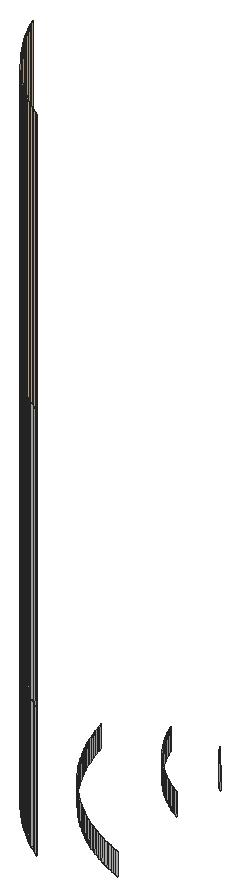
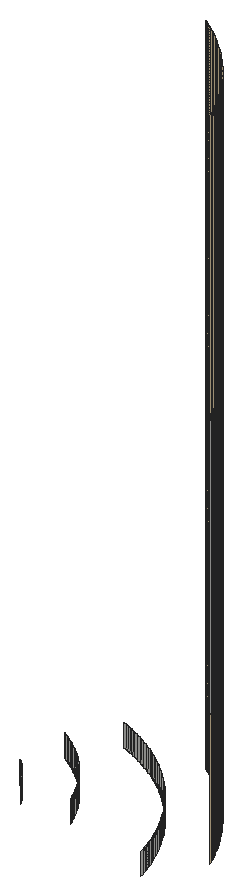
# SketchUp Ruby script. Lengths in inches.
U = 1.inch
M = Sketchup.active_model
def pt(a) = Geom::Point3d.new(a.map { |v| v * U })
def face(e, loops, mat)
  f = e.add_face(loops[0].map { |a| pt(a) })
  loops[1..].each { |l| e.add_face(l.map { |a| pt(a) }).erase! }
  f.material = f.back_material = mat if mat
  f
end
# faces: each face lists its corners as indices into pts; further lists are holes
def faces(e, pts, list, mat = nil) = list.each { |f| face(e, (f[0].is_a?(Array) ? f : [f]).map { |l| l.map { |i| pts[i] } }, mat) }
# xy, xz, yz: faces in a plane at the given z, y or x. An outline is a flat list of corners, or four numbers for a rectangle; further outlines are holes
def ring(l) = l.size == 4 ? [[l[0], l[1]], [l[2], l[1]], [l[2], l[3]], [l[0], l[3]]] : l.each_slice(2).to_a
def flat(e, list, mat, &to3) = list.each { |f| face(e, (f[0].is_a?(Array) ? f : [f]).map { |l| ring(l).map { |u, v| to3.(u, v) } }, mat) }
def xy(e, z, list, mat = nil) = flat(e, list, mat) { |x, y| [x, y, z] }
def xz(e, y, list, mat = nil) = flat(e, list, mat) { |x, z| [x, y, z] }
def yz(e, x, list, mat = nil) = flat(e, list, mat) { |y, z| [x, y, z] }
def lines(e, pts, list) = list.each { |a, b| e.add_line(pt(pts[a]), pt(pts[b])) }
# prism: a flat outline (further loops are holes) pulled along v
def prism(e, loops, v, mat = nil)
  f = face(e, loops, mat); d = Geom::Vector3d.new(v.map { |x| x * U })
  f.pushpull(f.normal.samedirection?(d) ? d.length : -d.length)
end
def box(e, o, s, mat = nil) = prism(e, [[o, [o[0] + s[0], o[1], o[2]], [o[0] + s[0], o[1] + s[1], o[2]], [o[0], o[1] + s[1], o[2]]]], [0, 0, s[2]], mat)
def at(x, y, z, deg = 0) = Geom::Transformation.translation(pt([x, y, z])) * Geom::Transformation.rotation(ORIGIN, Z_AXIS, deg.degrees)
def axes(o, x, y, z) = Geom::Transformation.new([*x, 0, *y, 0, *z, 0, *pt(o).to_a, 1])
def part(name) = M.definitions.add(name)
# library, detail: a bought-in or finely detailed component or shape, given as its bounding box
def library(name, o, s) = part(name).tap { |d| box(d.entities, o, s) }
def detail(e, o, s) = box(e.add_group.entities, o, s)
def put(e, d, t, mat = nil) = e.add_instance(d, t).tap { |i| i.material = mat if mat }
def group(e, t, mat = nil) = e.add_group.tap { |g| g.transformation = t; g.material = mat if mat }.entities
root = M.entities
M.materials.add("1026 AP 7946 SUNNY SIDE UP").color = [254, 231, 186]
p = [[23.33,229.02,252],[23.2,229.11,252],[23.2,229.11,246],[23.33,229.02,246],[23.36,229,246],[23.25,229.08,246],
  [23.25,229.08,276],[23.36,229,276],[23.15,229.15,246],[23.05,229.22,246],[23.05,229.22,276],[23.15,229.15,276],
  [23.07,229.2,252],[23.07,229.2,246],[22.95,229.29,246],[22.95,229.29,276],[22.95,229.29,252],[22.95,229.29,246],
  [22.85,229.37,246],[22.85,229.37,276],[22.82,229.38,252],[22.82,229.38,246],[22.74,229.44,246],[22.65,229.52,246],
  [22.65,229.52,276],[22.74,229.44,276],[22.69,229.48,252],[22.69,229.48,246],[22.55,229.6,246],[22.55,229.6,276],
  [22.57,229.58,252],[22.57,229.58,246],[22.45,229.67,246],[22.45,229.67,276],[22.45,229.67,252],[22.45,229.67,246],
  [26.54,229.62,246],[26.42,229.66,246],[26.42,229.66,247],[26.54,229.62,247],[22.33,229.77,252],[22.33,229.77,246],
  [22.35,229.75,246],[22.35,229.75,276],[26.29,229.71,246],[26.17,229.76,246],[26.17,229.76,247],[26.29,229.71,247],
  [22.25,229.83,246],[22.16,229.92,246],[22.16,229.92,276],[22.25,229.83,276],[22.21,229.875,252],[22.21,229.875,246],
  [26.05,229.8125,246],[25.93,229.86,246],[25.93,229.86,247],[26.05,229.8125,247],[22.0625,230,246],[22.0625,230,276],
  [22.09,229.98,252],[22.09,229.98,246],[25.8125,229.92,246],[25.69,229.97,246],[25.69,229.97,247],[25.8125,229.92,247],
  [21.97,230.08,246],[21.97,230.08,276],[21.97,230.08,252],[21.97,230.08,246],[25.58,230.03,246],[25.46,230.09,246],
  [25.46,230.09,247],[25.58,230.03,247],[21.88,230.17,246],[21.88,230.17,276],[21.85,230.1875,252],[21.85,230.1875,246],
  [25.34,230.15,246],[25.34,230.15,247],[21.74,230.3,252],[21.74,230.3,246],[21.79,230.25,246],[21.79,230.25,276],
  [25.23,230.21,246],[25.11,230.28,246],[25.11,230.28,247],[25.23,230.21,247],[21.69,230.34,246],[21.6,230.43,246],
  [21.6,230.43,276],[21.69,230.34,276],[21.625,230.4,252],[21.625,230.4,246],[25,230.34,246],[24.89,230.41,246],
  [24.89,230.41,247],[25,230.34,247],[21.51,230.51,246],[21.51,230.51,276],[21.51,230.51,252],[21.51,230.51,246],
  [24.78,230.47,246],[24.78,230.47,247],[21.43,230.6,246],[21.43,230.6,276],[21.4,230.625,252],[21.4,230.625,246],
  [24.66,230.54,246],[24.55,230.61,246],[24.55,230.61,247],[24.66,230.54,247],[21.34,230.69,246],[21.34,230.69,276],
  [21.3,230.74,252],[21.3,230.74,246],[24.44,230.69,246],[24.44,230.69,247],[21.1875,230.85,252],[21.1875,230.85,246],
  [21.25,230.79,246],[21.25,230.79,276],[24.34,230.76,246],[24.34,230.76,247],[21.17,230.88,246],[21.17,230.88,276],
  [24.23,230.83,246],[24.12,230.91,246],[24.12,230.91,247],[24.23,230.83,247],[21.08,230.97,246],[21.08,230.97,276],
  [21.08,230.97,252],[21.08,230.97,246],[24.02,230.99,246],[24.02,230.99,247],[21,231.0625,246],[21,231.0625,276],
  [20.98,231.09,252],[20.98,231.09,246],[23.91,231.07,246],[23.91,231.07,247],[20.92,231.16,246],[20.92,231.16,276],
  [20.875,231.21,252],[20.875,231.21,246],[23.81,231.15,246],[23.71,231.23,246],[23.71,231.23,247],[23.81,231.15,247],
  [20.83,231.25,246],[20.83,231.25,276],[20.77,231.33,252],[20.77,231.33,246],[23.61,231.3125,246],[23.61,231.3125,247],
  [20.67,231.45,252],[20.67,231.45,246],[20.75,231.35,246],[20.75,231.35,276],[23.51,231.4,246],[23.51,231.4,247],
  [20.67,231.45,246],[20.6,231.55,246],[20.6,231.55,276],[20.67,231.45,276],[20.58,231.57,252],[20.58,231.57,246],
  [23.41,231.48,246],[23.41,231.48,247],[20.52,231.65,246],[20.52,231.65,276],[23.31,231.57,246],[23.31,231.57,247],
  [20.44,231.74,246],[20.44,231.74,276],[20.48,231.69,252],[20.48,231.69,246],[23.21,231.66,246],[23.21,231.66,247],
  [20.37,231.85,246],[20.37,231.85,276],[20.38,231.82,252],[20.38,231.82,246],[23.12,231.75,246],[23.02,231.84,246],
  [23.02,231.84,247],[23.12,231.75,247],[20.29,231.95,246],[20.29,231.95,276],[20.29,231.95,252],[20.29,231.95,246],
  [22.93,231.93,246],[22.93,231.93,247],[20.22,232.05,246],[20.22,232.05,276],[20.2,232.07,252],[20.2,232.07,246],
  [22.84,232.02,246],[22.84,232.02,247],[20.15,232.15,246],[20.15,232.15,276],[22.75,232.12,246],[22.75,232.12,247],
  [20.11,232.2,252],[20.11,232.2,246],[22.66,232.21,246],[22.66,232.21,247],[20.02,232.33,252],[20.02,232.33,246],
  [20.08,232.25,246],[20.08,232.25,276],[22.57,232.31,246],[22.57,232.31,247],[19.9375,232.46,252],[19.9375,232.46,246],
  [20,232.36,246],[20,232.36,276],[22.48,232.41,246],[22.48,232.41,247],[19.9375,232.46,246],[19.9375,232.46,276],
  [22.4,232.51,246],[22.4,232.51,247],[19.87,232.57,246],[19.87,232.57,276],[19.85,232.6,252],[19.85,232.6,246],
  [22.3125,232.61,246],[22.3125,232.61,247],[19.8,232.68,246],[19.8,232.68,276],[19.77,232.73,252],[19.77,232.73,246],
  [22.23,232.71,246],[22.23,232.71,247],[19.74,232.78,246],[19.74,232.78,276],[19.6875,232.86,252],[19.6875,232.86,246],
  [22.15,232.81,246],[22.15,232.81,247],[19.67,232.89,246],[19.67,232.89,276],[22.07,232.91,246],[22.07,232.91,247],
  [19.61,233,246],[19.61,233,276],[19.61,233,252],[19.61,233,246],[21.99,233.02,246],[21.99,233.02,247],
  [19.55,233.11,246],[19.55,233.11,276],[19.53,233.14,252],[19.53,233.14,246],[21.91,233.12,246],[21.91,233.12,247],
  [19.48,233.22,246],[19.48,233.22,276],[19.45,233.27,252],[19.45,233.27,246],[21.83,233.23,246],[21.83,233.23,247],
  [19.42,233.33,246],[19.42,233.33,276],[21.76,233.34,246],[21.76,233.34,247],[19.37,233.44,246],[19.37,233.44,276],
  [19.38,233.41,252],[19.38,233.41,246],[21.69,233.44,246],[21.69,233.44,247],[19.31,233.55,246],[19.31,233.55,276],
  [19.31,233.55,252],[19.31,233.55,246],[21.61,233.55,246],[21.61,233.55,247],[19.24,233.69,252],[19.24,233.69,246],
  [19.25,233.66,246],[19.25,233.66,276],[21.54,233.66,246],[21.54,233.66,247],[19.2,233.78,246],[19.2,233.78,276],
  [19.17,233.83,252],[19.17,233.83,246],[21.47,233.78,246],[21.47,233.78,247],[19.14,233.89,246],[19.14,233.89,276],
  [19.1,233.98,252],[19.1,233.98,246],[21.41,233.89,246],[21.41,233.89,247],[19.09,234,246],[19.09,234,276],
  [21.34,234,246],[21.34,234,247],[19.04,234.12,246],[19.04,234.12,276],[19.04,234.12,252],[19.04,234.12,246],
  [21.28,234.11,246],[21.28,234.11,247],[18.99,234.23,246],[18.99,234.23,276],[21.21,234.23,246],[21.21,234.23,247],
  [21.15,234.34,246],[21.15,234.34,247],[21.09,234.46,246],[21.09,234.46,247],[21.03,234.58,246],[21.03,234.58,247],
  [20.97,234.69,246],[20.97,234.69,247],[20.92,234.8125,246],[20.92,234.8125,247],[20.86,234.93,246],[20.86,234.93,247],
  [20.8125,235.05,246],[20.8125,235.05,247],[20.76,235.17,246],[20.76,235.17,247],[20.71,235.29,246],[20.71,235.29,247],
  [20.66,235.42,246],[20.66,235.42,247],[20.62,235.54,246],[20.62,235.54,247],[20.57,235.66,246],[20.57,235.66,247],
  [20.53,235.79,246],[20.53,235.79,247],[20.49,235.91,246],[20.49,235.91,247],[20.45,236.03,246],[20.45,236.03,247],
  [20.41,236.16,246],[20.41,236.16,247],[20.375,236.29,246],[20.375,236.29,247],[20.34,236.41,246],[20.34,236.41,247],
  [26.5,232.9375,248],[26.5,232.9375,247],[26.42,232.98,247],[26.42,232.98,248],[26.58,232.89,248],[26.58,232.89,247],
  [26.34,233.03,248],[26.34,233.03,247],[26.26,233.08,247],[26.26,233.08,248],[26.1875,233.13,248],[26.1875,233.13,247],
  [26.11,233.18,247],[26.11,233.18,248],[26.04,233.23,248],[26.04,233.23,247],[25.96,233.28,247],[25.96,233.28,248],
  [25.89,233.34,248],[25.89,233.34,247],[25.8125,233.39,247],[25.8125,233.39,248],[25.74,233.45,248],[25.74,233.45,247],
  [25.67,233.5,247],[25.67,233.5,248],[25.59,233.56,247],[25.59,233.56,248],[25.52,233.62,248],[25.52,233.62,247],
  [25.45,233.68,247],[25.45,233.68,248],[25.38,233.74,248],[25.38,233.74,247],[25.32,233.8,247],[25.32,233.8,248],
  [25.25,233.86,247],[25.25,233.86,248],[25.18,233.92,248],[25.18,233.92,247],[25.12,233.99,247],[25.12,233.99,248],
  [25.05,234.05,247],[25.05,234.05,248],[24.99,234.12,248],[24.99,234.12,247],[24.92,234.18,247],[24.92,234.18,248],
  [24.86,234.25,248],[24.86,234.25,247],[24.8,234.32,247],[24.8,234.32,248],[24.74,234.38,247],[24.74,234.38,248],
  [24.68,234.45,247],[24.68,234.45,248],[24.62,234.52,248],[24.62,234.52,247],[24.56,234.59,247],[24.56,234.59,248],
  [24.5,234.67,247],[24.5,234.67,248],[24.45,234.74,248],[24.45,234.74,247],[24.39,234.8125,247],[24.39,234.8125,248],
  [24.34,234.89,247],[24.34,234.89,248],[24.28,234.96,247],[24.28,234.96,248],[24.23,235.04,248],[24.23,235.04,247],
  [24.18,235.11,247],[24.18,235.11,248],[24.13,235.1875,247],[24.13,235.1875,248],[24.08,235.26,247],[24.08,235.26,248],
  [24.03,235.34,248],[24.03,235.34,247],[23.98,235.42,247],[23.98,235.42,248],[26.56,235.375,247],[26.61,235.33,247],
  [26.61,235.33,248],[26.56,235.375,248],[23.9375,235.5,247],[23.9375,235.5,248],[26.46,235.46,247],[26.51,235.42,247],
  [26.51,235.42,248],[26.46,235.46,248],[23.89,235.58,247],[23.89,235.58,248],[26.375,235.56,247],[26.42,235.51,247],
  [26.42,235.51,248],[26.375,235.56,248],[23.85,235.66,247],[23.85,235.66,248],[26.28,235.65,247],[26.33,235.61,247],
  [26.33,235.61,248],[26.28,235.65,248],[23.81,235.74,248],[23.81,235.74,247],[23.76,235.82,247],[23.76,235.82,248],
  [26.2,235.75,247],[26.24,235.7,247],[26.24,235.7,248],[26.2,235.75,248],[23.72,235.9,247],[23.72,235.9,248],
  [26.11,235.85,247],[26.16,235.8,247],[26.16,235.8,248],[26.11,235.85,248],[23.68,235.99,247],[23.68,235.99,248],
  [26.03,235.96,247],[26.07,235.9,247],[26.07,235.9,248],[26.03,235.96,248],[23.64,236.07,247],[23.64,236.07,248],
  [25.95,236.0625,247],[25.99,236.01,247],[25.99,236.01,248],[25.95,236.0625,248],[23.61,236.15,247],[23.61,236.15,248],
  [25.88,236.17,247],[25.92,236.11,247],[25.92,236.11,248],[25.88,236.17,248],[23.57,236.24,248],[23.57,236.24,247],
  [23.53,236.32,247],[23.53,236.32,248],[25.81,236.28,247],[25.84,236.22,247],[25.84,236.22,248],[25.81,236.28,248],
  [23.5,236.41,247],[23.5,236.41,248],[25.74,236.39,247],[25.77,236.33,247],[25.77,236.33,248],[25.74,236.39,248],
  [25.7,236.44,247],[25.7,236.44,248],[23.33,229.02,264],[23.2,229.11,264],[23.2,229.11,252],[23.33,229.02,252],
  [23.07,229.2,264],[23.07,229.2,252],[22.95,229.29,264],[22.95,229.29,252],[22.82,229.38,264],[22.82,229.38,252],
  [22.69,229.48,264],[22.69,229.48,252],[22.57,229.58,264],[22.57,229.58,252],[22.45,229.67,264],[22.45,229.67,252],
  [22.33,229.77,264],[22.33,229.77,252],[22.21,229.875,264],[22.21,229.875,252],[22.09,229.98,264],[22.09,229.98,252],
  [21.97,230.08,264],[21.97,230.08,252],[21.85,230.1875,264],[21.85,230.1875,252],[21.74,230.3,264],[21.74,230.3,252],
  [21.625,230.4,264],[21.625,230.4,252],[21.51,230.51,264],[21.51,230.51,252],[21.4,230.625,264],[21.4,230.625,252],
  [21.3,230.74,264],[21.3,230.74,252],[21.1875,230.85,264],[21.1875,230.85,252],[21.08,230.97,264],[21.08,230.97,252],
  [20.98,231.09,264],[20.98,231.09,252],[20.875,231.21,264],[20.875,231.21,252],[20.77,231.33,264],[20.77,231.33,252],
  [20.67,231.45,264],[20.67,231.45,252],[20.58,231.57,264],[20.58,231.57,252],[20.48,231.69,264],[20.48,231.69,252],
  [20.38,231.82,264],[20.38,231.82,252],[20.29,231.95,264],[20.29,231.95,252],[20.2,232.07,264],[20.2,232.07,252],
  [20.11,232.2,264],[20.11,232.2,252],[20.02,232.33,264],[20.02,232.33,252],[19.9375,232.46,264],[19.9375,232.46,252],
  [19.85,232.6,264],[19.85,232.6,252],[19.77,232.73,264],[19.77,232.73,252],[19.6875,232.86,264],[19.6875,232.86,252],
  [19.61,233,264],[19.61,233,252],[19.53,233.14,264],[19.53,233.14,252],[19.45,233.27,264],[19.45,233.27,252],
  [19.38,233.41,264],[19.38,233.41,252],[19.31,233.55,264],[19.31,233.55,252],[19.24,233.69,264],[19.24,233.69,252],
  [19.17,233.83,264],[19.17,233.83,252],[19.1,233.98,264],[19.1,233.98,252],[19.04,234.12,264],[19.04,234.12,252],
  [18.97,234.26,264],[18.97,234.26,252]]
faces(root,p,[[0,1,2,3],[1,12,13,2],[12,16,17,13],[16,20,21,17],[20,26,27,21],[26,30,31,27],[30,34,35,31],[36,37,38,39],
  [34,40,41,35],[44,45,46,47],[37,44,47,38],[40,52,53,41],[54,55,56,57],[45,54,57,46],[52,60,61,53],[62,63,64,65],
  [55,62,65,56],[60,68,69,61],[70,71,72,73],[63,70,73,64],[68,76,77,69],[71,78,79,72],[76,80,81,77],[84,85,86,87],
  [78,84,87,79],[80,92,93,81],[94,95,96,97],[85,94,97,86],[92,100,101,93],[95,102,103,96],[100,106,107,101],[108,109,110,111],
  [102,108,111,103],[106,114,115,107],[109,116,117,110],[114,118,119,115],[116,122,123,117],[126,127,128,129],[122,126,129,123],[118,132,133,119],
  [127,134,135,128],[132,138,139,133],[134,140,141,135],[138,144,145,139],[146,147,148,149],[140,146,149,141],[144,152,153,145],[147,154,155,148],
  [152,156,157,153],[154,160,161,155],[156,166,167,157],[160,168,169,161],[168,172,173,169],[166,176,177,167],[172,178,179,173],[176,182,183,177],
  [184,185,186,187],[178,184,187,179],[182,190,191,183],[185,192,193,186],[190,196,197,191],[192,198,199,193],[198,202,203,199],[196,204,205,197],
  [202,206,207,203],[204,208,209,205],[206,212,213,207],[208,214,215,209],[212,218,219,213],[218,222,223,219],[214,226,227,215],[222,228,229,223],
  [226,232,233,227],[228,234,235,229],[232,238,239,233],[234,240,241,235],[240,244,245,241],[238,248,249,239],[244,250,251,245],[248,254,255,249],
  [250,256,257,251],[254,260,261,255],[256,262,263,257],[262,266,267,263],[260,270,271,261],[266,272,273,267],[270,276,277,271],[272,278,279,273],
  [276,280,281,277],[278,284,285,279],[280,288,289,281],[284,290,291,285],[288,294,295,289],[290,296,297,291],[296,300,301,297],[294,304,305,295],
  [300,306,307,301],[306,310,311,307],[310,312,313,311],[312,314,315,313],[314,316,317,315],[316,318,319,317],[318,320,321,319],[320,322,323,321],
  [322,324,325,323],[324,326,327,325],[326,328,329,327],[328,330,331,329],[330,332,333,331],[332,334,335,333],[334,336,337,335],[336,338,339,337],
  [338,340,341,339],[340,342,343,341],[342,344,345,343],[344,346,347,345],[348,349,350,351],[352,353,349,348],[354,355,356,357],[351,350,355,354],
  [358,359,360,361],[357,356,359,358],[362,363,364,365],[361,360,363,362],[366,367,368,369],[365,364,367,366],[370,371,372,373],[369,368,371,370],
  [373,372,374,375],[376,377,378,379],[375,374,377,376],[380,381,382,383],[379,378,381,380],[383,382,384,385],[386,387,388,389],[385,384,387,386],
  [389,388,390,391],[392,393,394,395],[391,390,393,392],[396,397,398,399],[395,394,397,396],[399,398,400,401],[401,400,402,403],[404,405,406,407],
  [403,402,405,404],[407,406,408,409],[410,411,412,413],[409,408,411,410],[413,412,414,415],[415,414,416,417],[418,419,420,421],[417,416,419,418],
  [421,420,422,423],[423,422,424,425],[426,427,428,429],[425,424,427,426],[430,431,432,433],[429,428,434,435],[436,437,438,439],[437,430,433,438],
  [435,434,440,441],[442,443,444,445],[443,436,439,444],[441,440,446,447],[448,449,450,451],[449,442,445,450],[452,453,454,455],[447,446,453,452],
  [456,457,458,459],[457,448,451,458],[455,454,460,461],[462,463,464,465],[463,456,459,464],[461,460,466,467],[468,469,470,471],[469,462,465,470],
  [467,466,472,473],[474,475,476,477],[475,468,471,476],[473,472,478,479],[480,481,482,483],[481,474,477,482],[484,485,486,487],[479,478,485,484],
  [488,489,490,491],[489,480,483,490],[487,486,492,493],[494,495,496,497],[495,488,491,496],[498,494,497,499],[500,501,502,503],[501,504,505,502],
  [504,506,507,505],[506,508,509,507],[508,510,511,509],[510,512,513,511],[512,514,515,513],[514,516,517,515],[516,518,519,517],[518,520,521,519],
  [520,522,523,521],[522,524,525,523],[524,526,527,525],[526,528,529,527],[528,530,531,529],[530,532,533,531],[532,534,535,533],[534,536,537,535],
  [536,538,539,537],[538,540,541,539],[540,542,543,541],[542,544,545,543],[544,546,547,545],[546,548,549,547],[548,550,551,549],[550,552,553,551],
  [552,554,555,553],[554,556,557,555],[556,558,559,557],[558,560,561,559],[560,562,563,561],[562,564,565,563],[564,566,567,565],[566,568,569,567],
  [568,570,571,569],[570,572,573,571],[572,574,575,573],[574,576,577,575],[576,578,579,577],[578,580,581,579],[580,582,583,581],[582,584,585,583],
  [584,586,587,585],[586,588,589,587]])
faces(root,p,[[4,5,6,7],[8,9,10,11],[5,8,11,6],[9,14,15,10],[14,18,19,15],[22,23,24,25],[18,22,25,19],[23,28,29,24],
  [28,32,33,29],[32,42,43,33],[48,49,50,51],[42,48,51,43],[49,58,59,50],[58,66,67,59],[66,74,75,67],[74,82,83,75],
  [88,89,90,91],[82,88,91,83],[89,98,99,90],[98,104,105,99],[104,112,113,105],[112,120,121,113],[120,124,125,121],[124,130,131,125],
  [130,136,137,131],[136,142,143,137],[142,150,151,143],[150,158,159,151],[162,163,164,165],[158,162,165,159],[163,170,171,164],[170,174,175,171],
  [174,180,181,175],[180,188,189,181],[188,194,195,189],[194,200,201,195],[200,210,211,201],[210,216,217,211],[216,220,221,217],[220,224,225,221],
  [224,230,231,225],[230,236,237,231],[236,242,243,237],[242,246,247,243],[246,252,253,247],[252,258,259,253],[258,264,265,259],[264,268,269,265],
  [268,274,275,269],[274,282,283,275],[282,286,287,283],[286,292,293,287],[292,298,299,293],[298,302,303,299],[302,308,309,303]],"1026 AP 7946 SUNNY SIDE UP")
